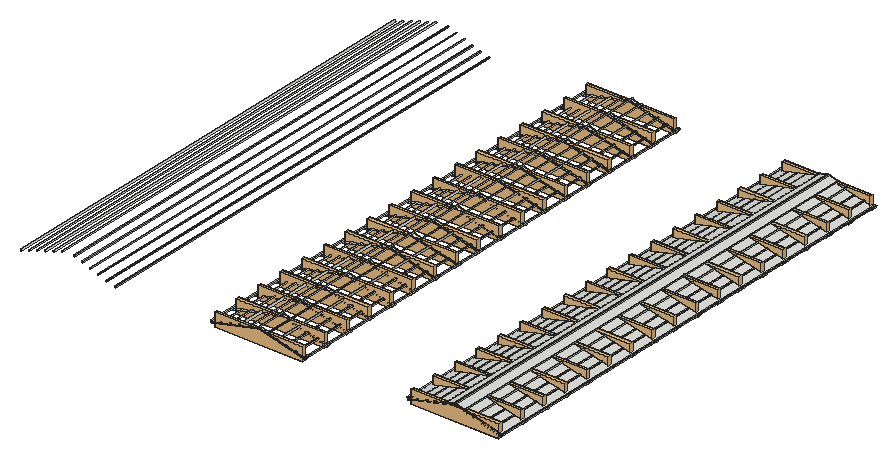
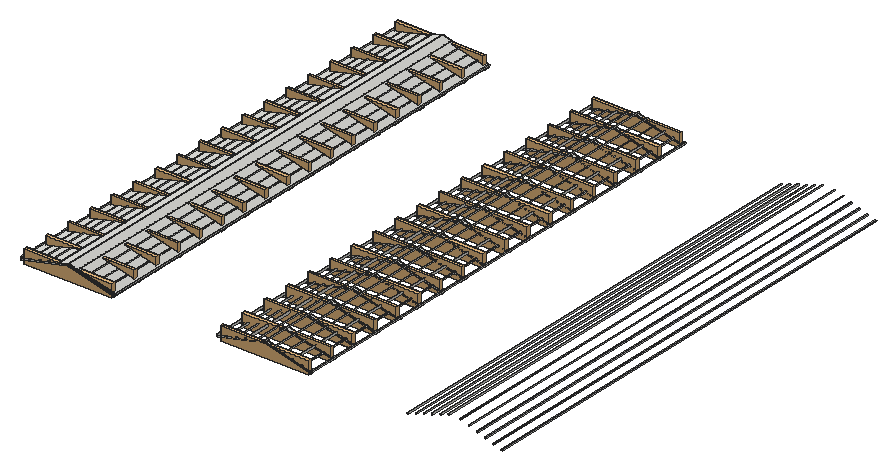
# SketchUp Ruby script. Lengths in inches.
U = 1.inch
M = Sketchup.active_model
def pt(a) = Geom::Point3d.new(a.map { |v| v * U })
def face(e, loops, mat)
  f = e.add_face(loops[0].map { |a| pt(a) })
  loops[1..].each { |l| e.add_face(l.map { |a| pt(a) }).erase! }
  f.material = f.back_material = mat if mat
  f
end
# faces: each face lists its corners as indices into pts; further lists are holes
def faces(e, pts, list, mat = nil) = list.each { |f| face(e, (f[0].is_a?(Array) ? f : [f]).map { |l| l.map { |i| pts[i] } }, mat) }
# xy, xz, yz: faces in a plane at the given z, y or x. An outline is a flat list of corners, or four numbers for a rectangle; further outlines are holes
def ring(l) = l.size == 4 ? [[l[0], l[1]], [l[2], l[1]], [l[2], l[3]], [l[0], l[3]]] : l.each_slice(2).to_a
def flat(e, list, mat, &to3) = list.each { |f| face(e, (f[0].is_a?(Array) ? f : [f]).map { |l| ring(l).map { |u, v| to3.(u, v) } }, mat) }
def xy(e, z, list, mat = nil) = flat(e, list, mat) { |x, y| [x, y, z] }
def xz(e, y, list, mat = nil) = flat(e, list, mat) { |x, z| [x, y, z] }
def yz(e, x, list, mat = nil) = flat(e, list, mat) { |y, z| [x, y, z] }
def lines(e, pts, list) = list.each { |a, b| e.add_line(pt(pts[a]), pt(pts[b])) }
# prism: a flat outline (further loops are holes) pulled along v
def prism(e, loops, v, mat = nil)
  f = face(e, loops, mat); d = Geom::Vector3d.new(v.map { |x| x * U })
  f.pushpull(f.normal.samedirection?(d) ? d.length : -d.length)
end
def box(e, o, s, mat = nil) = prism(e, [[o, [o[0] + s[0], o[1], o[2]], [o[0] + s[0], o[1] + s[1], o[2]], [o[0], o[1] + s[1], o[2]]]], [0, 0, s[2]], mat)
def at(x, y, z, deg = 0) = Geom::Transformation.translation(pt([x, y, z])) * Geom::Transformation.rotation(ORIGIN, Z_AXIS, deg.degrees)
def axes(o, x, y, z) = Geom::Transformation.new([*x, 0, *y, 0, *z, 0, *pt(o).to_a, 1])
def part(name) = M.definitions.add(name)
# library, detail: a bought-in or finely detailed component or shape, given as its bounding box
def library(name, o, s) = part(name).tap { |d| box(d.entities, o, s) }
def detail(e, o, s) = box(e.add_group.entities, o, s)
def put(e, d, t, mat = nil) = e.add_instance(d, t).tap { |i| i.material = mat if mat }
def group(e, t, mat = nil) = e.add_group.tap { |g| g.transformation = t; g.material = mat if mat }.entities
root = M.entities
c1 = library("Group\#9",[0,0,0],[492,18,73.96])
c2 = part("Group\#8")
xz(c2.entities,0,[[1.33,0,264,59.7,262.67,60,264,65.85,0,5.85],[526.67,0,528,5.85,264,65.85,265.33,60,264,59.7],[264,59.7,262.67,60,264,65.85,265.33,60]])
xz(c2.entities,18,[[1.33,0,0,5.85,264,65.85,262.67,60,264,59.7],[526.67,0,528,5.85,264,65.85,265.33,60,264,59.7],[264,59.7,265.33,60,264,65.85,262.67,60]])
p = [[0,0,5.85],[0,18,5.85],[1.33,18,0],[1.33,0,0],[264,18,59.7],[265.33,18,60],
  [265.33,0,60],[264,0,59.7],[526.67,18,0],[262.67,18,60],[262.67,0,60],[526.67,0,0],
  [528,0,5.85],[528,18,5.85],[264,0,65.85],[264,18,65.85]]
faces(c2.entities,p,[[0,1,2,3],[3,2,4,5,6,7],[8,4,9,10,7,11],[12,13,8,11],[1,0,14,15],[14,12,13,15],[15,14,10,9],[15,14,6,5]])
c3 = part("Group\#10")
prism(c3.entities,[[[106.64,0,23.94],[112.49,0,25.26],[111.17,0,31.12],[105.3125,0,29.79]]],[0,2602.6875,0])
prism(c3.entities,[[[159.3,0,35.9],[165.15,0,37.23],[163.82,0,43.08],[157.97,0,41.75]]],[0,2602.6875,0])
prism(c3.entities,[[[211.96,0,47.87],[217.81,0,49.2],[216.48,0,55.05],[210.63,0,53.72]]],[0,2602.6875,0])
prism(c3.entities,[[[476.67,0,11.97],[476.67,2602.6875,11.97],[478,2602.6875,17.82],[478,0,17.82]]],[-5.85,0,1.33])
prism(c3.entities,[[[418.16,0,25.26],[424.02,0,23.94],[425.35,0,29.79],[419.49,0,31.12]]],[0,2602.6875,0])
prism(c3.entities,[[[365.51,0,37.23],[371.36,0,35.9],[372.6875,0,41.75],[366.84,0,43.08]]],[0,2602.6875,0])
prism(c3.entities,[[[7.18,2602.6875,1.33],[1.33,2602.6875,0],[0,2602.6875,5.85],[5.85,2602.6875,7.18]]],[0,-2602.6875,0])
prism(c3.entities,[[[523.48,0,1.33],[529.33,0,0],[530.66,0,5.85],[524.81,0,7.18]]],[0,2602.6875,0])
prism(c3.entities,[[[312.85,0,49.2],[318.7,0,47.87],[320.03,0,53.72],[314.18,0,55.05]]],[0,2602.6875,0])
prism(c3.entities,[[[266.04,2602.6875,59.84],[260.19,2602.6875,61.17],[261.52,2602.6875,67.02],[267.375,2602.6875,65.6875]]],[0,-2602.6875,0])
prism(c3.entities,[[[59.84,2602.6875,13.3],[53.99,2602.6875,11.97],[52.66,2602.6875,17.82],[58.51,2602.6875,19.15]]],[0,-2602.6875,0])
prism(root,[[[2417.45,0,275.02],[2155.93,0,213.85],[2155.93,2602.6875,213.85],[2417.45,2602.6875,275.02]]],[-0.23,0,0.97])
xz(root,0,[[2686.59,213.85,2686.81,214.83,2423.52,274.66,2423.3,273.6875]])
p = [[2423.3,0,273.6875],[2423.3,2602.6875,273.6875],[2686.59,2601.5625,213.85],[2686.59,0,213.85],[2686.81,2601.5625,214.83],[2686.81,2599.39,214.83],
  [2686.81,2597.43,214.83],[2686.81,2588.55,214.83],[2686.81,2586.4,214.83],[2686.81,2584.43,214.83],[2686.81,2575.54,214.83],[2686.81,2573.4,214.83],
  [2686.81,2571.43,214.83],[2686.81,2562.52,214.83],[2686.81,2560.4,214.83],[2686.81,2558.43,214.83],[2686.81,2549.51,214.83],[2686.81,2547.4,214.83],
  [2686.81,2545.4375,214.83],[2686.81,2536.5,214.83],[2686.81,2534.41,214.83],[2686.81,2532.4375,214.83],[2686.81,2523.48,214.83],[2686.81,2521.41,214.83],
  [2686.81,2519.44,214.83],[2686.81,2510.47,214.83],[2686.81,2508.41,214.83],[2686.81,2506.44,214.83],[2686.81,2497.46,214.83],[2686.81,2495.41,214.83],
  [2686.81,2493.45,214.83],[2686.81,2484.44,214.83],[2686.81,2482.42,214.83],[2686.81,2480.45,214.83],[2686.81,2471.43,214.83],[2686.81,2469.42,214.83],
  [2686.81,2467.45,214.83],[2686.81,2458.41,214.83],[2686.81,2456.42,214.83],[2686.81,2454.45,214.83],[2686.81,2445.4,214.83],[2686.81,2443.42,214.83],
  [2686.81,2441.46,214.83],[2686.81,2432.39,214.83],[2686.81,2430.43,214.83],[2686.81,2428.46,214.83],[2686.81,2419.375,214.83],[2686.81,2417.43,214.83],
  [2686.81,2415.46,214.83],[2686.81,2406.36,214.83],[2686.81,2404.43,214.83],[2686.81,2402.46,214.83],[2686.81,2393.35,214.83],[2686.81,2391.43,214.83],
  [2686.81,2389.47,214.83],[2686.81,2380.33,214.83],[2686.81,2378.4375,214.83],[2686.81,2376.47,214.83],[2686.81,2367.32,214.83],[2686.81,2365.44,214.83],
  [2686.81,2363.47,214.83],[2686.81,2354.31,214.83],[2686.81,2352.44,214.83],[2686.81,2350.47,214.83],[2686.81,2341.29,214.83],[2686.81,2339.44,214.83],
  [2686.81,2337.48,214.83],[2686.81,2328.28,214.83],[2686.81,2326.45,214.83],[2686.81,2324.48,214.83],[2686.81,2315.27,214.83],[2686.81,2313.45,214.83],
  [2686.81,2311.48,214.83],[2686.81,2302.25,214.83],[2686.81,2300.45,214.83],[2686.81,2298.48,214.83],[2686.81,2289.24,214.83],[2686.81,2287.45,214.83],
  [2686.81,2285.49,214.83],[2686.81,2276.23,214.83],[2686.81,2274.46,214.83],[2686.81,2272.49,214.83],[2686.81,2263.21,214.83],[2686.81,2261.46,214.83],
  [2686.81,2259.49,214.83],[2686.81,2250.2,214.83],[2686.81,2248.46,214.83],[2686.81,2246.49,214.83],[2686.81,2237.1875,214.83],[2686.81,2235.46,214.83],
  [2686.81,2233.5,214.83],[2686.81,2224.17,214.83],[2686.81,2222.47,214.83],[2686.81,2220.5,214.83],[2686.81,2211.16,214.83],[2686.81,2209.47,214.83],
  [2686.81,2207.5,214.83],[2686.81,2198.15,214.83],[2686.81,2196.47,214.83],[2686.81,2194.5,214.83],[2686.81,2185.13,214.83],[2686.81,2183.47,214.83],
  [2686.81,2181.51,214.83],[2686.81,2172.12,214.83],[2686.81,2170.48,214.83],[2686.81,2168.51,214.83],[2686.81,2159.11,214.83],[2686.81,2157.48,214.83],
  [2686.81,2155.51,214.83],[2686.81,2146.09,214.83],[2686.81,2144.48,214.83],[2686.81,2142.51,214.83],[2686.81,2133.08,214.83],[2686.81,2131.48,214.83],
  [2686.81,2129.52,214.83],[2686.81,2120.07,214.83],[2686.81,2118.49,214.83],[2686.81,2116.52,214.83],[2686.81,2107.05,214.83],[2686.81,2105.49,214.83],
  [2686.81,2103.52,214.83],[2686.81,2094.04,214.83],[2686.81,2092.49,214.83],[2686.81,2090.52,214.83],[2686.81,2081.03,214.83],[2686.81,2079.49,214.83],
  [2686.81,2077.53,214.83],[2686.81,2068.01,214.83],[2686.81,2066.5,214.83],[2686.81,2064.53,214.83],[2686.81,2055,214.83],[2686.81,2053.5,214.83],
  [2686.81,2051.53,214.83],[2686.81,2041.98,214.83],[2686.81,2040.5,214.83],[2686.81,2038.53,214.83],[2686.81,2028.97,214.83],[2686.81,2027.5,214.83],
  [2686.81,2025.54,214.83],[2686.81,2015.96,214.83],[2686.81,2014.51,214.83],[2686.81,2012.54,214.83],[2686.81,2002.94,214.83],[2686.81,2001.51,214.83],
  [2686.81,1999.54,214.83],[2686.81,1989.93,214.83],[2686.81,1988.51,214.83],[2686.81,1986.54,214.83],[2686.81,1976.92,214.83],[2686.81,1975.51,214.83],
  [2686.81,1973.55,214.83],[2686.81,1963.9,214.83],[2686.81,1962.52,214.83],[2686.81,1960.55,214.83],[2686.81,1950.89,214.83],[2686.81,1949.52,214.83],
  [2686.81,1947.55,214.83],[2686.81,1937.88,214.83],[2686.81,1936.52,214.83],[2686.81,1934.55,214.83],[2686.81,1924.86,214.83],[2686.81,1923.52,214.83],
  [2686.81,1921.56,214.83],[2686.81,1911.85,214.83],[2686.81,1910.53,214.83],[2686.81,1908.56,214.83],[2686.81,1898.84,214.83],[2686.81,1897.53,214.83],
  [2686.81,1895.5625,214.83],[2686.81,1885.82,214.83],[2686.81,1884.53,214.83],[2686.81,1882.5625,214.83],[2686.81,1872.81,214.83],[2686.81,1871.53,214.83],
  [2686.81,1869.57,214.83],[2686.81,1859.8,214.83],[2686.81,1858.54,214.83],[2686.81,1856.57,214.83],[2686.81,1846.78,214.83],[2686.81,1845.54,214.83],
  [2686.81,1843.57,214.83],[2686.81,1833.77,214.83],[2686.81,1832.54,214.83],[2686.81,1830.57,214.83],[2686.81,1820.76,214.83],[2686.81,1819.54,214.83],
  [2686.81,1817.58,214.83],[2686.81,1807.74,214.83],[2686.81,1806.55,214.83],[2686.81,1804.58,214.83],[2686.81,1794.73,214.83],[2686.81,1793.55,214.83],
  [2686.81,1791.58,214.83],[2686.81,1781.72,214.83],[2686.81,1780.55,214.83],[2686.81,1778.58,214.83],[2686.81,1768.7,214.83],[2686.81,1767.55,214.83],
  [2686.81,1765.59,214.83],[2686.81,1755.6875,214.83],[2686.81,1754.56,214.83],[2686.81,1752.59,214.83],[2686.81,1742.68,214.83],[2686.81,1741.56,214.83],
  [2686.81,1739.59,214.83],[2686.81,1729.66,214.83],[2686.81,1728.5625,214.83],[2686.81,1726.59,214.83],[2686.81,1716.65,214.83],[2686.81,1715.5625,214.83],
  [2686.81,1713.6,214.83],[2686.81,1703.64,214.83],[2686.81,1702.57,214.83],[2686.81,1700.6,214.83],[2686.81,1690.62,214.83],[2686.81,1689.57,214.83],
  [2686.81,1687.6,214.83],[2686.81,1677.61,214.83],[2686.81,1676.57,214.83],[2686.81,1674.6,214.83],[2686.81,1664.6,214.83],[2686.81,1663.57,214.83],
  [2686.81,1661.61,214.83],[2686.81,1651.58,214.83],[2686.81,1650.58,214.83],[2686.81,1648.61,214.83],[2686.81,1638.57,214.83],[2686.81,1637.58,214.83],
  [2686.81,1635.61,214.83],[2686.81,1625.55,214.83],[2686.81,1624.58,214.83],[2686.81,1622.61,214.83],[2686.81,1612.54,214.83],[2686.81,1611.58,214.83],
  [2686.81,1609.62,214.83],[2686.81,1599.53,214.83],[2686.81,1598.59,214.83],[2686.81,1596.62,214.83],[2686.81,1586.51,214.83],[2686.81,1585.59,214.83],
  [2686.81,1583.62,214.83],[2686.81,1573.5,214.83],[2686.81,1572.59,214.83],[2686.81,1570.62,214.83],[2686.81,1560.49,214.83],[2686.81,1559.59,214.83],
  [2686.81,1557.625,214.83],[2686.81,1547.47,214.83],[2686.81,1546.6,214.83],[2686.81,1544.63,214.83],[2686.81,1534.46,214.83],[2686.81,1533.6,214.83],
  [2686.81,1531.63,214.83],[2686.81,1521.45,214.83],[2686.81,1520.6,214.83],[2686.81,1518.63,214.83],[2686.81,1508.43,214.83],[2686.81,1507.6,214.83],
  [2686.81,1505.64,214.83],[2686.81,1495.42,214.83],[2686.81,1492.64,214.83],[2686.81,1482.41,214.83],[2686.81,1479.64,214.83],[2686.81,1469.39,214.83],
  [2686.81,1466.64,214.83],[2686.81,1456.38,214.83],[2686.81,1453.65,214.83],[2686.81,1443.37,214.83],[2686.81,1440.65,214.83],[2686.81,1430.35,214.83],
  [2686.81,1427.65,214.83],[2686.81,1417.34,214.83],[2686.81,1414.65,214.83],[2686.81,1404.33,214.83],[2686.81,1401.65,214.83],[2686.81,1391.3125,214.83],
  [2686.81,1388.66,214.83],[2686.81,1378.3,214.83],[2686.81,1375.66,214.83],[2686.81,1365.29,214.83],[2686.81,1362.66,214.83],[2686.81,1352.27,214.83],
  [2686.81,1349.66,214.83],[2686.81,1339.26,214.83],[2686.81,1336.67,214.83],[2686.81,1326.25,214.83],[2686.81,1323.67,214.83],[2686.81,1313.23,214.83],
  [2686.81,1310.67,214.83],[2686.81,1300.22,214.83],[2686.81,1297.67,214.83],[2686.81,1287.21,214.83],[2686.81,1284.68,214.83],[2686.81,1274.19,214.83],
  [2686.81,1271.68,214.83],[2686.81,1261.18,214.83],[2686.81,1258.68,214.83],[2686.81,1248.16,214.83],[2686.81,1245.68,214.83],[2686.81,1235.15,214.83],
  [2686.81,1232.6875,214.83],[2686.81,1222.14,214.83],[2686.81,1219.69,214.83],[2686.81,1209.125,214.83],[2686.81,1206.69,214.83],[2686.81,1196.11,214.83],
  [2686.81,1193.69,214.83],[2686.81,1183.1,214.83],[2686.81,1180.7,214.83],[2686.81,1170.08,214.83],[2686.81,1167.7,214.83],[2686.81,1157.07,214.83],
  [2686.81,1154.7,214.83],[2686.81,1144.06,214.83],[2686.81,1141.7,214.83],[2686.81,1131.04,214.83],[2686.81,1128.71,214.83],[2686.81,1118.03,214.83],
  [2686.81,1115.71,214.83],[2686.81,1105.02,214.83],[2686.81,1102.71,214.83],[2686.81,1092,214.83],[2686.81,1089.71,214.83],[2686.81,1078.99,214.83],
  [2686.81,1076.72,214.83],[2686.81,1065.98,214.83],[2686.81,1063.72,214.83],[2686.81,1052.96,214.83],[2686.81,1050.72,214.83],[2686.81,1039.95,214.83],
  [2686.81,1037.72,214.83],[2686.81,1026.9375,214.83],[2686.81,1024.73,214.83],[2686.81,1013.92,214.83],[2686.81,1011.73,214.83],[2686.81,1000.91,214.83],
  [2686.81,998.73,214.83],[2686.81,987.9,214.83],[2686.81,985.73,214.83],[2686.81,974.88,214.83],[2686.81,972.74,214.83],[2686.81,961.87,214.83],
  [2686.81,959.74,214.83],[2686.81,948.86,214.83],[2686.81,946.74,214.83],[2686.81,935.84,214.83],[2686.81,933.74,214.83],[2686.81,922.83,214.83],
  [2686.81,920.75,214.83],[2686.81,909.82,214.83],[2686.81,907.75,214.83],[2686.81,896.8,214.83],[2686.81,894.75,214.83],[2686.81,883.79,214.83],
  [2686.81,881.75,214.83],[2686.81,870.78,214.83],[2686.81,868.76,214.83],[2686.81,857.76,214.83],[2686.81,855.76,214.83],[2686.81,844.75,214.83],
  [2686.81,842.76,214.83],[2686.81,831.73,214.83],[2686.81,829.76,214.83],[2686.81,818.73,214.83],[2686.81,816.77,214.83],[2686.81,805.74,214.83],
  [2686.81,803.77,214.83],[2686.81,792.74,214.83],[2686.81,790.77,214.83],[2686.81,779.74,214.83],[2686.81,777.77,214.83],[2686.81,766.74,214.83],
  [2686.81,764.78,214.83],[2686.81,753.75,214.83],[2686.81,751.78,214.83],[2686.81,740.75,214.83],[2686.81,738.78,214.83],[2686.81,727.75,214.83],
  [2686.81,725.78,214.83],[2686.81,714.75,214.83],[2686.81,712.79,214.83],[2686.81,701.76,214.83],[2686.81,699.79,214.83],[2686.81,688.76,214.83],
  [2686.81,686.79,214.83],[2686.81,675.76,214.83],[2686.81,673.79,214.83],[2686.81,662.76,214.83],[2686.81,660.8,214.83],[2686.81,649.77,214.83],
  [2686.81,647.8,214.83],[2686.81,636.77,214.83],[2686.81,634.8,214.83],[2686.81,623.77,214.83],[2686.81,621.8,214.83],[2686.81,610.77,214.83],
  [2686.81,608.81,214.83],[2686.81,597.78,214.83],[2686.81,595.81,214.83],[2686.81,584.78,214.83],[2686.81,582.8125,214.83],[2686.81,571.78,214.83],
  [2686.81,569.8125,214.83],[2686.81,558.78,214.83],[2686.81,556.82,214.83],[2686.81,545.79,214.83],[2686.81,543.82,214.83],[2686.81,532.79,214.83],
  [2686.81,530.82,214.83],[2686.81,519.79,214.83],[2686.81,517.82,214.83],[2686.81,506.79,214.83],[2686.81,504.83,214.83],[2686.81,493.8,214.83],
  [2686.81,491.83,214.83],[2686.81,480.8,214.83],[2686.81,478.83,214.83],[2686.81,467.8,214.83],[2686.81,465.83,214.83],[2686.81,454.8,214.83],
  [2686.81,452.84,214.83],[2686.81,441.81,214.83],[2686.81,439.84,214.83],[2686.81,428.81,214.83],[2686.81,426.84,214.83],[2686.81,415.8125,214.83],
  [2686.81,413.84,214.83],[2686.81,402.8125,214.83],[2686.81,400.85,214.83],[2686.81,389.82,214.83],[2686.81,387.85,214.83],[2686.81,376.82,214.83],
  [2686.81,374.85,214.83],[2686.81,363.82,214.83],[2686.81,361.85,214.83],[2686.81,350.82,214.83],[2686.81,348.86,214.83],[2686.81,337.83,214.83],
  [2686.81,335.86,214.83],[2686.81,324.83,214.83],[2686.81,322.86,214.83],[2686.81,311.83,214.83],[2686.81,309.86,214.83],[2686.81,298.83,214.83],
  [2686.81,296.87,214.83],[2686.81,285.84,214.83],[2686.81,283.87,214.83],[2686.81,272.84,214.83],[2686.81,270.87,214.83],[2686.81,259.84,214.83],
  [2686.81,257.875,214.83],[2686.81,246.84,214.83],[2686.81,244.875,214.83],[2686.81,233.85,214.83],[2686.81,231.88,214.83],[2686.81,220.85,214.83],
  [2686.81,218.88,214.83],[2686.81,207.85,214.83],[2686.81,205.88,214.83],[2686.81,194.85,214.83],[2686.81,192.89,214.83],[2686.81,181.86,214.83],
  [2686.81,179.89,214.83],[2686.81,168.86,214.83],[2686.81,166.89,214.83],[2686.81,155.86,214.83],[2686.81,153.89,214.83],[2686.81,142.86,214.83],
  [2686.81,140.9,214.83],[2686.81,129.87,214.83],[2686.81,127.9,214.83],[2686.81,116.87,214.83],[2686.81,114.9,214.83],[2686.81,103.87,214.83],
  [2686.81,101.9,214.83],[2686.81,90.875,214.83],[2686.81,88.91,214.83],[2686.81,77.875,214.83],[2686.81,75.91,214.83],[2686.81,64.88,214.83],
  [2686.81,62.91,214.83],[2686.81,51.88,214.83],[2686.81,49.91,214.83],[2686.81,38.88,214.83],[2686.81,36.92,214.83],[2686.81,25.89,214.83],
  [2686.81,23.92,214.83],[2686.81,12.89,214.83],[2686.81,10.92,214.83],[2686.81,0,214.83],[2423.52,2602.6875,274.66]]
faces(root,p,[[0,1,2,3],[3,2,4,5,6,7,8,9,10,11,12,13,14,15,16,17,18,19,20,21,22,23,24,25,26,27,28,29,30,31,32,33,34,35,36,37,38,39,40,41,42,43,44,45,46,47,48,49,50,51,52,53,54,55,56,57,58,59,60,61,62,63,64,65,66,67,68,69,70,71,72,73,74,75,76,77,78,79,80,81,82,83,84,85,86,87,88,89,90,91,92,93,94,95,96,97,98,99,100,101,102,103,104,105,106,107,108,109,110,111,112,113,114,115,116,117,118,119,120,121,122,123,124,125,126,127,128,129,130,131,132,133,134,135,136,137,138,139,140,141,142,143,144,145,146,147,148,149,150,151,152,153,154,155,156,157,158,159,160,161,162,163,164,165,166,167,168,169,170,171,172,173,174,175,176,177,178,179,180,181,182,183,184,185,186,187,188,189,190,191,192,193,194,195,196,197,198,199,200,201,202,203,204,205,206,207,208,209,210,211,212,213,214,215,216,217,218,219,220,221,222,223,224,225,226,227,228,229,230,231,232,233,234,235,236,237,238,239,240,241,242,243,244,245,246,247,248,249,250,251,252,253,254,255,256,257,258,259,260,261,262,263,264,265,266,267,268,269,270,271,272,273,274,275,276,277,278,279,280,281,282,283,284,285,286,287,288,289,290,291,292,293,294,295,296,297,298,299,300,301,302,303,304,305,306,307,308,309,310,311,312,313,314,315,316,317,318,319,320,321,322,323,324,325,326,327,328,329,330,331,332,333,334,335,336,337,338,339,340,341,342,343,344,345,346,347,348,349,350,351,352,353,354,355,356,357,358,359,360,361,362,363,364,365,366,367,368,369,370,371,372,373,374,375,376,377,378,379,380,381,382,383,384,385,386,387,388,389,390,391,392,393,394,395,396,397,398,399,400,401,402,403,404,405,406,407,408,409,410,411,412,413,414,415,416,417,418,419,420,421,422,423,424,425,426,427,428,429,430,431,432,433,434,435,436,437,438,439,440,441,442,443,444,445,446,447,448,449,450,451,452,453,454,455,456,457,458,459,460,461,462,463,464,465,466,467,468,469,470,471,472,473,474,475,476,477,478,479,480,481,482,483,484,485,486,487,488,489],[2,1,490,4]])
put(root,c1,at(1080.94,0,187.9))
put(root,c1,at(1080.94,152,187.9))
put(root,c1,at(1080.94,304,187.9))
put(root,c1,at(1080.94,456,187.9))
put(root,c1,at(1080.94,608,187.9))
put(root,c1,at(1080.94,760,187.9))
put(root,c1,at(1080.94,912,187.9))
put(root,c1,at(1080.94,1064,187.9))
put(root,c1,at(1080.94,1216,187.9))
put(root,c1,at(1080.94,1368,187.9))
put(root,c1,at(1080.94,1520,187.9))
put(root,c1,at(1080.94,1672,187.9))
put(root,c1,at(1080.94,1824,187.9))
put(root,c1,at(1080.94,1976,187.9))
put(root,c1,at(1080.94,2128,187.9))
put(root,c1,at(1080.94,2280,187.9))
put(root,c1,at(1080.94,2432,187.9))
put(root,c1,at(1080.94,2584,187.9))
put(root,c1,at(2175.26,456,187.9))
put(root,c1,at(2175.26,2584,187.9))
put(root,c1,at(2175.26,152,187.9))
put(root,c1,at(2175.26,760,187.9))
put(root,c1,at(2175.26,2128,187.9))
put(root,c1,at(2175.26,912,187.9))
put(root,c1,at(2175.26,0,187.9))
put(root,c1,at(2175.26,1976,187.9))
put(root,c1,at(2175.26,304,187.9))
put(root,c1,at(2175.26,608,187.9))
put(root,c1,at(2175.26,1824,187.9))
put(root,c1,at(2175.26,1520,187.9))
put(root,c1,at(2175.26,2280,187.9))
put(root,c1,at(2175.26,1672,187.9))
put(root,c1,at(2175.26,1064,187.9))
put(root,c1,at(2175.26,1216,187.9))
put(root,c1,at(2175.26,2432,187.9))
put(root,c1,at(2175.26,1368,187.9))
g1 = group(root,at(0,0,190))
prism(g1,[[[478.36,0,16.37],[484.08,0,14.55],[485.9,0,20.27],[480.18,0,22.09]]],[0,2602,0])
prism(g1,[[[529.82,2602,0],[524.1,2602,1.82],[525.92,2602,7.54],[531.64,2602,5.72]]],[0,-2602,0])
prism(g1,[[[139.04,2602,43.66],[139.04,0,43.66],[137.22,0,49.38],[137.22,2602,49.38]]],[5.72,0,1.82])
prism(g1,[[[93.3,2602,29.11],[93.3,0,29.11],[91.48,0,34.83],[91.48,2602,34.83]]],[5.72,0,1.82])
prism(g1,[[[1.82,0,0],[7.54,0,1.82],[5.72,0,7.54],[0,0,5.72]]],[0,2602,0])
prism(g1,[[[190.5,0,60.03],[184.78,0,58.22],[184.78,2602,58.22],[190.5,2602,60.03]]],[-1.82,0,5.72])
prism(g1,[[[236.24,0,74.59],[230.52,0,72.77],[230.52,2602,72.77],[236.24,2602,74.59]]],[-1.82,0,5.72])
prism(g1,[[[346.86,2602,58.22],[341.14,2602,60.03],[342.96,2602,65.75],[348.68,2602,63.93]]],[0,-2602,0])
prism(g1,[[[392.6,2602,43.66],[386.88,2602,45.48],[388.7,2602,51.2],[394.42,2602,49.38]]],[0,-2602,0])
prism(g1,[[[53.28,0,16.37],[47.56,0,14.55],[47.56,2602,14.55],[53.28,2602,16.37]]],[-1.82,0,5.72])
prism(g1,[[[301.12,0,72.77],[301.12,2602,72.77],[302.9375,2602,78.49],[302.9375,0,78.49]]],[-5.72,0,1.82])
prism(g1,[[[438.34,2602,29.11],[432.62,2602,30.93],[434.44,2602,36.64],[440.16,2602,34.83]]],[0,-2602,0])
put(root,c2,at(1062.94,0,202.15))
put(root,c2,at(1062.94,152,202.15))
put(root,c2,at(1062.94,304,202.15))
put(root,c2,at(1062.94,456,202.15))
put(root,c2,at(1062.94,608,202.15))
put(root,c2,at(1062.94,760,202.15))
put(root,c2,at(1062.94,912,202.15))
put(root,c2,at(1062.94,1064,202.15))
put(root,c2,at(1062.94,1216,202.15))
put(root,c2,at(1062.94,1368,202.15))
put(root,c2,at(1062.94,1520,202.15))
put(root,c2,at(1062.94,1672,202.15))
put(root,c2,at(1062.94,1824,202.15))
put(root,c2,at(1062.94,1976,202.15))
put(root,c2,at(1062.94,2128,202.15))
put(root,c2,at(1062.94,2280,202.15))
put(root,c2,at(1062.94,2432,202.15))
put(root,c2,at(1062.94,2584,202.15))
put(root,c2,at(2157.26,304,202.15))
put(root,c2,at(2157.26,2584,202.15))
put(root,c2,at(2157.26,1672,202.15))
put(root,c2,at(2157.26,2280,202.15))
put(root,c2,at(2157.26,0,202.15))
put(root,c2,at(2157.26,608,202.15))
put(root,c2,at(2157.26,456,202.15))
put(root,c2,at(2157.26,1368,202.15))
put(root,c2,at(2157.26,2432,202.15))
put(root,c2,at(2157.26,1824,202.15))
put(root,c2,at(2157.26,152,202.15))
put(root,c2,at(2157.26,2128,202.15))
put(root,c2,at(2157.26,1520,202.15))
put(root,c2,at(2157.26,1216,202.15))
put(root,c2,at(2157.26,912,202.15))
put(root,c2,at(2157.26,1064,202.15))
put(root,c2,at(2157.26,1976,202.15))
put(root,c2,at(2157.26,760,202.15))
put(root,c3,at(1061.61,0,208))
put(root,c3,at(2155.93,0,208))
